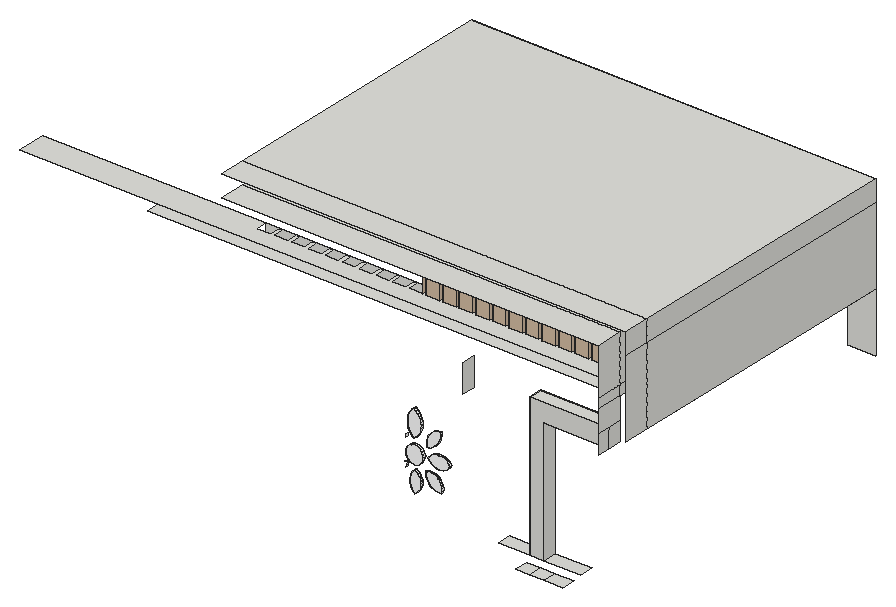
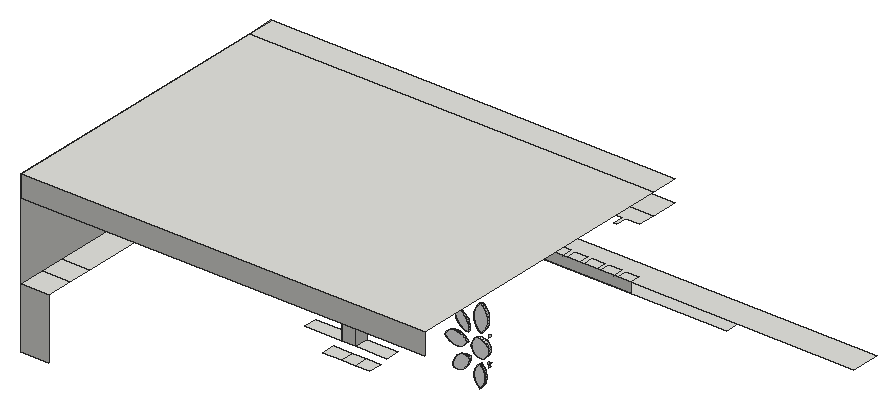
# SketchUp Ruby script. Lengths in inches.
U = 1.inch
M = Sketchup.active_model
def pt(a) = Geom::Point3d.new(a.map { |v| v * U })
def face(e, loops, mat)
  f = e.add_face(loops[0].map { |a| pt(a) })
  loops[1..].each { |l| e.add_face(l.map { |a| pt(a) }).erase! }
  f.material = f.back_material = mat if mat
  f
end
# faces: each face lists its corners as indices into pts; further lists are holes
def faces(e, pts, list, mat = nil) = list.each { |f| face(e, (f[0].is_a?(Array) ? f : [f]).map { |l| l.map { |i| pts[i] } }, mat) }
# xy, xz, yz: faces in a plane at the given z, y or x. An outline is a flat list of corners, or four numbers for a rectangle; further outlines are holes
def ring(l) = l.size == 4 ? [[l[0], l[1]], [l[2], l[1]], [l[2], l[3]], [l[0], l[3]]] : l.each_slice(2).to_a
def flat(e, list, mat, &to3) = list.each { |f| face(e, (f[0].is_a?(Array) ? f : [f]).map { |l| ring(l).map { |u, v| to3.(u, v) } }, mat) }
def xy(e, z, list, mat = nil) = flat(e, list, mat) { |x, y| [x, y, z] }
def xz(e, y, list, mat = nil) = flat(e, list, mat) { |x, z| [x, y, z] }
def yz(e, x, list, mat = nil) = flat(e, list, mat) { |y, z| [x, y, z] }
def lines(e, pts, list) = list.each { |a, b| e.add_line(pt(pts[a]), pt(pts[b])) }
# prism: a flat outline (further loops are holes) pulled along v
def prism(e, loops, v, mat = nil)
  f = face(e, loops, mat); d = Geom::Vector3d.new(v.map { |x| x * U })
  f.pushpull(f.normal.samedirection?(d) ? d.length : -d.length)
end
def box(e, o, s, mat = nil) = prism(e, [[o, [o[0] + s[0], o[1], o[2]], [o[0] + s[0], o[1] + s[1], o[2]], [o[0], o[1] + s[1], o[2]]]], [0, 0, s[2]], mat)
def at(x, y, z, deg = 0) = Geom::Transformation.translation(pt([x, y, z])) * Geom::Transformation.rotation(ORIGIN, Z_AXIS, deg.degrees)
def axes(o, x, y, z) = Geom::Transformation.new([*x, 0, *y, 0, *z, 0, *pt(o).to_a, 1])
def part(name) = M.definitions.add(name)
# library, detail: a bought-in or finely detailed component or shape, given as its bounding box
def library(name, o, s) = part(name).tap { |d| box(d.entities, o, s) }
def detail(e, o, s) = box(e.add_group.entities, o, s)
def put(e, d, t, mat = nil) = e.add_instance(d, t).tap { |i| i.material = mat if mat }
def group(e, t, mat = nil) = e.add_group.tap { |g| g.transformation = t; g.material = mat if mat }.entities
root = M.entities
M.materials.add("[Color M00]").color = [255, 255, 255]
M.materials.add("[Formica Laminate Light]").color = [213, 189, 164]
prism(root,[[[333.78,152.35,246.9375],[333.21,152.35,247.375],[332.78,152.35,247.95],[332.5,152.35,248.61],[332.41,152.35,249.32],[332.5,152.35,250.03],[332.78,152.35,250.7],[333.21,152.35,251.26],[333.78,152.35,251.7],[334.45,152.35,251.98],[335.16,152.35,252.07],[335.87,152.35,251.98],[336.53,152.35,251.7],[337.1,152.35,251.26],[337.54,152.35,250.7],[337.8125,152.35,250.03],[337.91,152.35,249.32],[337.8125,152.35,248.61],[337.54,152.35,247.95],[337.1,152.35,247.375],[336.53,152.35,246.9375],[335.87,152.35,246.66],[335.16,152.35,246.57],[334.45,152.35,246.66]]],[0,-0.9375,0],"[Color M00]")
prism(root,[[[334.15,152.35,261.74],[334.77,152.35,262.29],[335.45,152.35,261.78],[336.03,152.35,261.16],[336.51,152.35,260.46],[336.85,152.35,259.68],[337.07,152.35,258.86],[337.14,152.35,258.01],[337.07,152.35,257.16],[336.85,152.35,256.34],[336.51,152.35,255.5625],[336.03,152.35,254.86],[335.45,152.35,254.24],[334.77,152.35,253.73],[334.15,152.35,254.28],[333.625,152.35,254.91],[333.2,152.35,255.62],[332.89,152.35,256.39],[332.7,152.35,257.1875],[332.64,152.35,258.01],[332.7,152.35,258.83],[332.89,152.35,259.64],[333.2,152.35,260.4],[333.625,152.35,261.11]]],[0,-0.5625,0],"[Color M00]")
prism(root,[[[339.2,151.79,245.81],[338.53,151.79,245.65],[338.52,151.79,245],[338.61,151.79,244.35],[338.8,151.79,243.72],[339.08,151.79,243.125],[339.45,151.79,242.58],[339.9,151.79,242.1],[340.41,151.79,241.7],[340.99,151.79,241.375],[341.6,151.79,241.15],[342.24,151.79,241.01],[342.9,151.79,240.98],[343.55,151.79,241.05],[343.65,151.79,241.73],[343.62,151.79,242.42],[343.48,151.79,243.09],[343.22,151.79,243.73],[342.85,151.79,244.31],[342.38,151.79,244.8125],[341.84,151.79,245.23],[341.23,151.79,245.55],[340.57,151.79,245.75],[339.89,151.79,245.84]]],[0,0.5625,0],"[Color M00]")
prism(root,[[[343.2,151.79,257.48],[343.16,151.79,258.19],[342.49,151.79,258.13],[341.83,151.79,257.98],[341.2,151.79,257.73],[340.62,151.79,257.39],[340.1,151.79,256.97],[339.64,151.79,256.47],[339.27,151.79,255.91],[338.98,151.79,255.3],[338.79,151.79,254.65],[338.7,151.79,253.99],[338.71,151.79,253.3125],[338.82,151.79,252.65],[339.52,151.79,252.78],[340.19,151.79,253.01],[340.82,151.79,253.33],[341.4,151.79,253.74],[341.92,151.79,254.24],[342.36,151.79,254.8],[342.71,151.79,255.41],[342.97,151.79,256.07],[343.14,151.79,256.77]]],[0,0.5625,0],"[Color M00]")
prism(root,[[[339.25,152.35,249.63],[339.62,152.35,250.2],[340.1,152.35,250.6875],[340.68,152.35,251.09],[341.33,152.35,251.39],[342.04,152.35,251.57],[342.77,152.35,251.63],[343.5,152.35,251.57],[344.2,152.35,251.39],[344.85,152.35,251.09],[345.43,152.35,250.6875],[345.91,152.35,250.2],[346.28,152.35,249.63],[345.91,152.35,249.07],[345.43,152.35,248.58],[344.85,152.35,248.18],[344.2,152.35,247.88],[343.5,152.35,247.7],[342.77,152.35,247.64],[342.04,152.35,247.7],[341.33,152.35,247.88],[340.68,152.35,248.18],[340.1,152.35,248.58],[339.62,152.35,249.07]]],[0,-0.5625,0],"[Color M00]")
xy(root,230.58,[[370.09,148.04,374.5,152.35],[374.5,148.04,379.09,152.35],[379.09,148.04,385.11,152.35]])
xy(root,236.1,[[364.57,148.04,374.5,152.35],[374.5,148.04,379.09,152.35],[379.09,148.04,390.63,152.35]])
xy(root,275.21,[[379.09,148.04,399.65,152.35]])
xy(root,281.1,[[374.5,148.04,399.65,152.35]])
xy(root,281.9375,[[399.27,161.35,408.27,226.93],[399.27,226.93,408.27,234.75],[399.27,234.75,408.27,243.33]])
xy(root,288.3125,[[249.72,152.35,399.65,161.35]])
xy(root,291.4375,[[209.34,152.35,399.65,152.35,399.65,157.85,396.14,157.85,396.14,161.35,395.2,161.35,395.2,157.85,391.58,157.85,391.58,161.35,390.63,161.35,390.63,157.85,386.27,157.85,386.27,161.35,385.38,161.35,385.38,157.85,381.02,157.85,381.02,161.35,380.13,161.35,380.13,157.85,375.77,157.85,375.77,161.35,374.88,161.35,374.88,157.85,370.52,157.85,370.52,161.35,369.63,161.35,369.63,157.85,365.27,157.85,365.27,161.35,364.38,161.35,364.38,157.85,360.02,157.85,360.02,161.35,359.13,161.35,359.13,157.85,354.77,157.85,354.77,161.35,353.88,161.35,353.88,157.85,349.52,157.85,349.52,161.35,348.63,161.35,348.63,157.85,344.27,157.85,344.27,161.35,343.38,161.35,343.38,157.85,339.02,157.85,339.02,161.35,338.13,161.35,338.13,157.85,333.77,157.85,333.77,161.35,332.76,161.35,332.76,157.85,328.39,157.85,328.39,161.35,327.38,161.35,327.38,157.85,323.02,157.85,323.02,161.35,322.01,161.35,322.01,157.85,317.64,157.85,317.64,161.35,316.63,161.35,316.63,157.85,312.27,157.85,312.27,161.35,311.26,161.35,311.26,157.85,306.89,157.85,306.89,161.35,305.88,161.35,305.88,157.85,301.52,157.85,301.52,161.35,300.51,161.35,300.51,157.85,296.14,157.85,296.14,161.35,295.13,161.35,295.13,157.85,290.77,157.85,290.77,161.35,289.76,161.35,289.76,157.85,285.39,157.85,285.39,161.35,284.38,161.35,284.38,157.85,280.02,157.85,280.02,161.35,209.34,161.35],[333.77,157.85,338.13,161.35],[339.02,157.85,343.38,161.35],[344.27,157.85,348.63,161.35],[349.52,157.85,353.88,161.35],
  [354.77,157.85,359.13,161.35],[360.02,157.85,364.38,161.35],[365.27,157.85,369.63,161.35],[370.52,157.85,374.88,161.35],[375.77,157.85,380.13,161.35],
  [381.02,157.85,385.38,161.35],[386.27,157.85,390.63,161.35],[391.58,157.85,395.2,161.35],[396.14,157.85,399.27,161.35],[399.27,157.85,399.65,161.35]])
xy(root,306.375,[[280.02,143.85,399.65,152.35],[280.02,152.35,280.02,157.85,284.38,157.85,284.38,161.35,285.39,161.35,285.39,157.85,289.76,157.85,289.76,161.35,290.77,161.35,290.77,157.85,295.13,157.85,295.13,161.35,296.14,161.35,296.14,157.85,300.51,157.85,300.51,161.35,301.52,161.35,301.52,157.85,305.88,157.85,305.88,161.35,306.89,161.35,306.89,157.85,311.26,157.85,311.26,161.35,312.27,161.35,312.27,157.85,316.63,157.85,316.63,161.35,317.64,161.35,317.64,157.85,322.01,157.85,322.01,161.35,323.02,161.35,323.02,157.85,327.38,157.85,327.38,161.35,328.39,161.35,328.39,157.85,332.76,157.85,332.76,161.35,333.77,161.35,333.77,157.85,338.13,157.85,338.13,161.35,339.02,161.35,339.02,157.85,343.38,157.85,343.38,161.35,344.27,161.35,344.27,157.85,348.63,157.85,348.63,161.35,349.52,161.35,349.52,157.85,353.88,157.85,353.88,161.35,354.77,161.35,354.77,157.85,359.13,157.85,359.13,161.35,360.02,161.35,360.02,157.85,364.38,157.85,364.38,161.35,365.27,161.35,365.27,157.85,369.63,157.85,369.63,161.35,370.52,161.35,370.52,157.85,374.88,157.85,374.88,161.35,375.77,161.35,375.77,157.85,380.13,157.85,380.13,161.35,381.02,161.35,381.02,157.85,385.38,157.85,385.38,161.35,386.27,161.35,386.27,157.85,390.63,157.85,390.63,161.35,391.58,161.35,391.58,157.85,395.2,157.85,395.2,161.35,396.14,161.35,396.14,157.85,399.65,157.85,399.65,152.35],[333.77,157.85,338.13,161.35],[339.02,157.85,343.38,161.35],[344.27,157.85,348.63,161.35],
  [349.52,157.85,353.88,161.35],[354.77,157.85,359.13,161.35],[360.02,157.85,364.38,161.35],[365.27,157.85,369.63,161.35],[370.52,157.85,374.88,161.35],
  [375.77,157.85,380.13,161.35],[381.02,157.85,385.38,161.35],[386.27,157.85,390.63,161.35],[391.58,157.85,395.2,161.35],[396.14,157.85,399.65,161.35]])
xy(root,313.1875,[[280.02,143.85,408.27,152.35],[280.02,152.35,408.27,243.33]])
xz(root,148.04,[[374.5,236.1,379.09,236.1,379.09,275.21,399.65,275.21,399.65,281.1,374.5,281.1]])
xz(root,151.79,[[335.02,238.02,335.59,238.43,336.08,238.92,336.48,239.49,336.77,240.11,336.94,240.77,337,241.45,336.94,242.13,336.77,242.8,336.48,243.42,336.08,243.99,335.59,244.48,335.02,244.88,334.5625,244.42,334.17,243.9,333.86,243.33,333.63,242.72,333.5,242.09,333.45,241.45,333.5,240.81,333.63,240.18,333.86,239.57,334.17,239.01,334.5625,238.48]],"[Color M00]")
xz(root,152.35,[[374.5,236.1,374.5,281.1,399.65,281.1,399.65,275.21,379.09,275.21,379.09,236.1]])
xz(root,152.35,[[335.02,238.02,334.5625,238.48,334.17,239.01,333.86,239.57,333.63,240.18,333.5,240.81,333.45,241.45,333.5,242.09,333.63,242.72,333.86,243.33,334.17,243.9,334.5625,244.42,335.02,244.88,335.59,244.48,336.08,243.99,336.48,243.42,336.77,242.8,336.94,242.13,337,241.45,336.94,240.77,336.77,240.11,336.48,239.49,336.08,238.92,335.59,238.43]],"[Color M00]")
xz(root,152.41,[[335.02,238.02,334.5625,238.48,334.17,239.01,333.86,239.57,333.63,240.18,333.5,240.81,333.45,241.45,333.5,242.09,333.63,242.72,333.86,243.33,334.17,243.9,334.5625,244.42,335.02,244.88,335.59,244.48,336.08,243.99,336.48,243.42,336.77,242.8,336.94,242.13,337,241.45,336.94,240.77,336.77,240.11,336.48,239.49,336.08,238.92,335.59,238.43]],"[Color M00]")
xz(root,157.85,[[333.77,291.4375,338.13,306.375],[339.02,291.4375,343.38,306.375],[344.27,291.4375,348.63,306.375],[349.52,291.4375,353.88,306.375],[354.77,291.4375,359.13,306.375],
  [360.02,291.4375,364.38,306.375],[365.27,291.4375,369.63,306.375],[370.52,291.4375,374.88,306.375],[375.77,291.4375,380.13,306.375],[381.02,291.4375,385.38,306.375],
  [386.27,291.4375,390.63,306.375],[391.58,291.4375,395.2,306.375],[396.14,291.4375,399.65,306.375]],"[Formica Laminate Light]")
xz(root,161.35,[[399.27,281.9375,399.65,288.3125],[280.02,288.3125,399.27,291.4375],[399.27,288.3125,399.65,291.4375],[332.76,291.4375,333.77,306.375],[333.77,291.4375,338.13,306.375],
  [338.13,291.4375,339.02,306.375],[339.02,291.4375,343.38,306.375],[343.38,291.4375,344.27,306.375],[344.27,291.4375,348.63,306.375],[348.63,291.4375,349.52,306.375],
  [349.52,291.4375,353.88,306.375],[353.88,291.4375,354.77,306.375],[354.77,291.4375,359.13,306.375],[359.13,291.4375,360.02,306.375],[360.02,291.4375,364.38,306.375],
  [364.38,291.4375,365.27,306.375],[365.27,291.4375,369.63,306.375],[369.63,291.4375,370.52,306.375],[370.52,291.4375,374.88,306.375],[374.88,291.4375,375.77,306.375],
  [375.77,291.4375,380.13,306.375],[380.13,291.4375,381.02,306.375],[381.02,291.4375,385.38,306.375],[385.38,291.4375,386.27,306.375],[386.27,291.4375,390.63,306.375],
  [390.63,291.4375,391.58,306.375],[391.58,291.4375,395.2,306.375],[395.2,291.4375,396.14,306.375],[396.14,291.4375,399.65,306.375]])
xz(root,243.33,[[399.27,262.6875,408.27,281.9375],[280.02,306.375,408.27,313.1875]])
yz(root,332.76,[[157.85,291.4375,161.35,306.375]],"[Formica Laminate Light]")
yz(root,333.77,[[157.85,291.4375,161.35,306.375]],"[Formica Laminate Light]")
yz(root,338.13,[[157.85,291.4375,161.35,306.375]],"[Formica Laminate Light]")
yz(root,339.02,[[157.85,291.4375,161.35,306.375]],"[Formica Laminate Light]")
yz(root,343.38,[[157.85,291.4375,161.35,306.375]],"[Formica Laminate Light]")
yz(root,344.27,[[157.85,291.4375,161.35,306.375]],"[Formica Laminate Light]")
yz(root,348.63,[[157.85,291.4375,161.35,306.375]],"[Formica Laminate Light]")
yz(root,349.52,[[157.85,291.4375,161.35,306.375]],"[Formica Laminate Light]")
yz(root,353.17,[[148.16,274.4,152.35,283.34]])
yz(root,353.88,[[157.85,291.4375,161.35,306.375]],"[Formica Laminate Light]")
yz(root,354.77,[[157.85,291.4375,161.35,306.375]],"[Formica Laminate Light]")
yz(root,359.13,[[157.85,291.4375,161.35,306.375]],"[Formica Laminate Light]")
yz(root,360.02,[[157.85,291.4375,161.35,306.375]],"[Formica Laminate Light]")
yz(root,364.38,[[157.85,291.4375,161.35,306.375]],"[Formica Laminate Light]")
yz(root,365.27,[[157.85,291.4375,161.35,306.375]],"[Formica Laminate Light]")
yz(root,369.63,[[157.85,291.4375,161.35,306.375]],"[Formica Laminate Light]")
yz(root,370.52,[[157.85,291.4375,161.35,306.375]],"[Formica Laminate Light]")
yz(root,374.5,[[148.04,236.1,152.35,281.1]])
yz(root,374.88,[[157.85,291.4375,161.35,306.375]],"[Formica Laminate Light]")
yz(root,375.77,[[157.85,291.4375,161.35,306.375]],"[Formica Laminate Light]")
yz(root,379.09,[[148.04,236.1,152.35,275.21]])
yz(root,380.13,[[157.85,291.4375,161.35,306.375]],"[Formica Laminate Light]")
yz(root,381.02,[[157.85,291.4375,161.35,306.375]],"[Formica Laminate Light]")
yz(root,385.38,[[157.85,291.4375,161.35,306.375]],"[Formica Laminate Light]")
yz(root,386.27,[[157.85,291.4375,161.35,306.375]],"[Formica Laminate Light]")
yz(root,390.63,[[157.85,291.4375,161.35,306.375]],"[Formica Laminate Light]")
yz(root,391.58,[[157.85,291.4375,161.35,306.375]],"[Formica Laminate Light]")
yz(root,395.2,[[157.85,291.4375,161.35,306.375]],"[Formica Laminate Light]")
yz(root,396.14,[[157.85,291.4375,161.35,306.375]],"[Formica Laminate Light]")
yz(root,399.65,[[143.85,275.21,148.04,281.1],[148.04,275.21,152.35,281.1],[143.85,281.1,152.35,288.3125],[143.85,288.3125,152.35,291.4375],[152.35,288.3125,161.35,291.4375],
  [143.85,291.4375,152.35,306.375],[152.35,291.4375,157.85,306.375],[157.85,291.4375,161.35,306.375]])
yz(root,408.27,[[143.85,281.9375,152.35,306.375],[152.35,281.9375,243.33,306.375],[143.85,306.375,152.35,313.1875],[152.35,306.375,243.33,313.1875]])
p = [[334.5625,152.35,238.48],[335.02,152.35,238.02],[335.02,151.79,238.02],[334.5625,151.79,238.48],[335.59,152.35,238.43],[335.59,151.79,238.43],
  [334.5625,152.41,238.48],[335.02,152.41,238.02],[335.59,152.41,238.43],[336.08,152.35,238.92],[336.08,151.79,238.92],[336.08,152.41,238.92],
  [334.17,152.35,239.01],[334.17,151.79,239.01],[334.17,152.41,239.01],[336.48,152.35,239.49],[336.48,151.79,239.49],[336.48,152.41,239.49],
  [333.86,152.35,239.57],[333.86,151.79,239.57],[333.86,152.41,239.57],[336.77,152.35,240.11],[336.77,151.79,240.11],[336.77,152.41,240.11],
  [333.63,152.35,240.18],[333.63,151.79,240.18],[333.63,152.41,240.18],[336.94,152.35,240.77],[336.94,151.79,240.77],[336.94,152.41,240.77],
  [333.5,152.35,240.81],[333.5,151.79,240.81],[333.5,152.41,240.81],[333.45,152.35,241.45],[333.45,151.79,241.45],[337,152.35,241.45],
  [337,151.79,241.45],[333.45,152.41,241.45],[337,152.41,241.45],[333.5,152.35,242.09],[333.5,151.79,242.09],[336.94,152.35,242.13],
  [336.94,151.79,242.13],[333.5,152.41,242.09],[336.94,152.41,242.13],[333.63,152.35,242.72],[333.63,151.79,242.72],[336.77,152.35,242.8],
  [336.77,151.79,242.8],[333.63,152.41,242.72],[336.77,152.41,242.8],[333.86,152.35,243.33],[333.86,151.79,243.33],[333.86,152.41,243.33],
  [336.48,152.35,243.42],[336.48,151.79,243.42],[336.48,152.41,243.42],[334.17,152.35,243.9],[334.17,151.79,243.9],[334.17,152.41,243.9],
  [336.08,152.35,243.99],[336.08,151.79,243.99],[336.08,152.41,243.99],[334.5625,152.35,244.42],[334.5625,151.79,244.42],[334.5625,152.41,244.42],
  [335.59,152.35,244.48],[335.59,151.79,244.48],[335.59,152.41,244.48],[335.02,152.35,244.88],[335.02,151.79,244.88],[335.02,152.41,244.88],
  [332.25,152.35,244.71],[332.5,152.35,245.4],[332.5,151.79,245.4],[332.25,151.79,244.71],[332.64,152.35,246.13],[332.64,151.79,246.13],
  [331.92,152.35,246.15],[331.92,151.79,246.15],[332.1875,152.35,253.33],[332.22,152.35,254.0625],[332.22,151.79,254.0625],[332.1875,151.79,253.33]]
faces(root,p,[[0,1,2,3],[1,4,5,2],[1,0,6,7],[4,1,7,8],[4,9,10,5],[9,4,8,11],[12,0,3,13],[0,12,14,6],
  [9,15,16,10],[15,9,11,17],[18,12,13,19],[12,18,20,14],[15,21,22,16],[21,15,17,23],[24,18,19,25],[18,24,26,20],
  [21,27,28,22],[27,21,23,29],[30,24,25,31],[24,30,32,26],[33,30,31,34],[27,35,36,28],[30,33,37,32],[35,27,29,38],
  [39,33,34,40],[35,41,42,36],[33,39,43,37],[41,35,38,44],[45,39,40,46],[41,47,48,42],[39,45,49,43],[47,41,44,50],
  [51,45,46,52],[45,51,53,49],[47,54,55,48],[54,47,50,56],[57,51,52,58],[51,57,59,53],[54,60,61,55],[60,54,56,62],
  [63,57,58,64],[57,63,65,59],[60,66,67,61],[66,60,62,68],[69,63,64,70],[63,69,71,65],[66,69,70,67],[69,66,68,71],
  [72,73,74,75],[73,76,77,74],[76,78,79,77],[80,81,82,83]],"[Color M00]")
